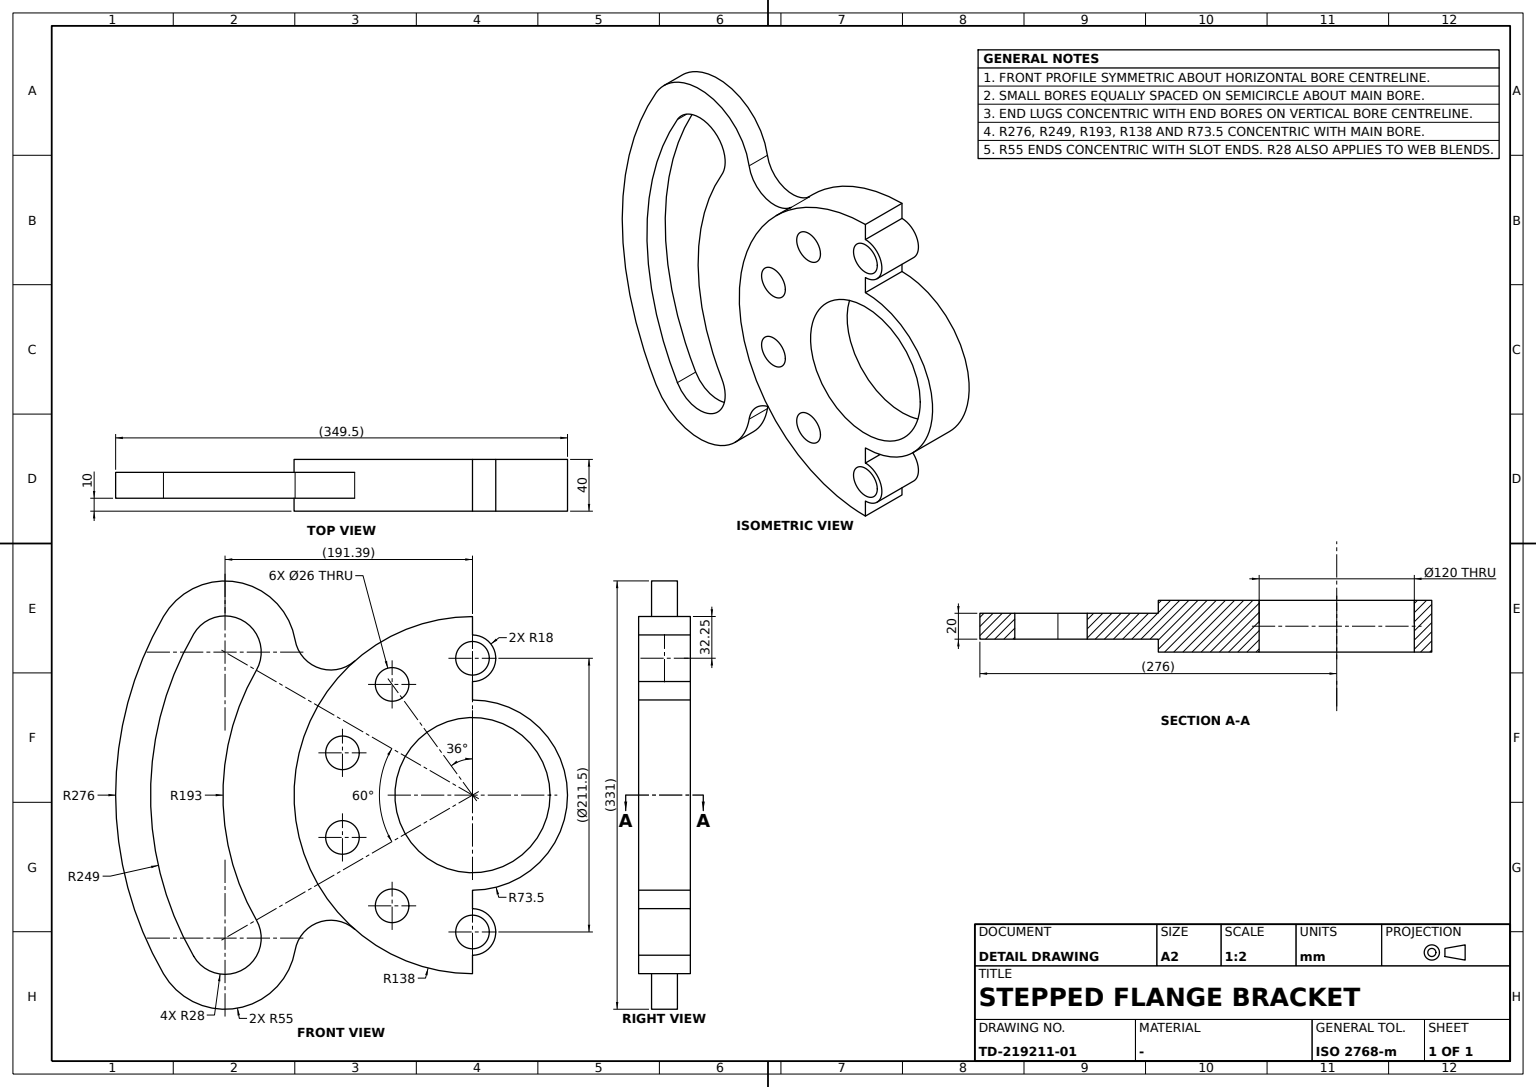
ISO-10303-21;
HEADER;
FILE_DESCRIPTION((''),'2;1');
FILE_NAME('','',(''),(''),'','','');
FILE_SCHEMA(('AUTOMOTIVE_DESIGN'));
ENDSEC;
DATA;
#1=APPLICATION_CONTEXT('');
#2=PRODUCT_CONTEXT('',#1,'mechanical');
#3=PRODUCT('','','',(#2));
#4=PRODUCT_DEFINITION_FORMATION('','',#3);
#5=PRODUCT_DEFINITION_CONTEXT('',#1,'design');
#6=PRODUCT_DEFINITION('','',#4,#5);
#7=PRODUCT_DEFINITION_SHAPE('','',#6);
#8=(LENGTH_UNIT()NAMED_UNIT(*)SI_UNIT(.MILLI.,.METRE.));
#9=(NAMED_UNIT(*)PLANE_ANGLE_UNIT()SI_UNIT($,.RADIAN.));
#10=(NAMED_UNIT(*)SI_UNIT($,.STERADIAN.)SOLID_ANGLE_UNIT());
#11=UNCERTAINTY_MEASURE_WITH_UNIT(LENGTH_MEASURE(0.005),#8,'distance_accuracy_value','');
#12=(GEOMETRIC_REPRESENTATION_CONTEXT(3)GLOBAL_UNCERTAINTY_ASSIGNED_CONTEXT((#11))GLOBAL_UNIT_ASSIGNED_CONTEXT((#8,#9,#10))REPRESENTATION_CONTEXT('',''));
#13=CARTESIAN_POINT('',(0.,-87.75,-20.));
#14=VERTEX_POINT('',#13);
#15=CARTESIAN_POINT('',(0.,-87.75,20.));
#16=VERTEX_POINT('',#15);
#17=DIRECTION('',(0.,0.,-1.));
#18=VECTOR('',#17,1000.);
#19=LINE('',#15,#18);
#20=EDGE_CURVE('',#14,#16,#19,.F.);
#21=ORIENTED_EDGE('',*,*,#20,.T.);
#22=CARTESIAN_POINT('',(0.,-123.75,20.));
#23=VERTEX_POINT('',#22);
#24=CARTESIAN_POINT('',(0.,-105.75,20.));
#25=DIRECTION('',(0.,0.,1.));
#26=DIRECTION('',(1.,0.,0.));
#27=AXIS2_PLACEMENT_3D('',#24,#25,#26);
#28=CIRCLE('',#27,18.);
#29=EDGE_CURVE('',#16,#23,#28,.F.);
#30=ORIENTED_EDGE('',*,*,#29,.T.);
#31=CARTESIAN_POINT('',(0.,-123.75,-20.));
#32=VERTEX_POINT('',#31);
#33=LINE('',#22,#18);
#34=EDGE_CURVE('',#23,#32,#33,.T.);
#35=ORIENTED_EDGE('',*,*,#34,.T.);
#36=CARTESIAN_POINT('',(0.,-105.75,-20.));
#37=AXIS2_PLACEMENT_3D('',#36,#25,#26);
#38=CIRCLE('',#37,18.);
#39=EDGE_CURVE('',#14,#32,#38,.F.);
#40=ORIENTED_EDGE('',*,*,#39,.F.);
#41=EDGE_LOOP('',(#21,#30,#35,#40));
#42=FACE_BOUND('',#41,.T.);
#43=CARTESIAN_POINT('',(0.,-105.75,0.));
#44=DIRECTION('',(0.,-1.,0.));
#45=AXIS2_PLACEMENT_3D('',#43,#17,#44);
#46=CYLINDRICAL_SURFACE('',#45,18.);
#47=ADVANCED_FACE('',(#42),#46,.T.);
#48=CARTESIAN_POINT('',(-215.640326,-124.5,10.));
#49=VERTEX_POINT('',#48);
#50=CARTESIAN_POINT('',(-215.640326,-124.5,-10.));
#51=VERTEX_POINT('',#50);
#52=CARTESIAN_POINT('',(-215.640326,-124.5,0.));
#53=VECTOR('',#25,1000.);
#54=LINE('',#52,#53);
#55=EDGE_CURVE('',#49,#51,#54,.F.);
#56=ORIENTED_EDGE('',*,*,#55,.F.);
#57=CARTESIAN_POINT('',(-167.142903,-96.5,10.));
#58=VERTEX_POINT('',#57);
#59=CARTESIAN_POINT('',(-191.391614,-110.5,10.));
#60=AXIS2_PLACEMENT_3D('',#59,#25,#26);
#61=CIRCLE('',#60,28.);
#62=EDGE_CURVE('',#49,#58,#61,.T.);
#63=ORIENTED_EDGE('',*,*,#62,.T.);
#64=CARTESIAN_POINT('',(-167.142903,-96.5,-10.));
#65=VERTEX_POINT('',#64);
#66=CARTESIAN_POINT('',(-167.142903,-96.5,0.));
#67=LINE('',#66,#53);
#68=EDGE_CURVE('',#58,#65,#67,.F.);
#69=ORIENTED_EDGE('',*,*,#68,.T.);
#70=CARTESIAN_POINT('',(-191.391614,-110.5,-10.));
#71=AXIS2_PLACEMENT_3D('',#70,#25,#26);
#72=CIRCLE('',#71,28.);
#73=EDGE_CURVE('',#51,#65,#72,.T.);
#74=ORIENTED_EDGE('',*,*,#73,.F.);
#75=EDGE_LOOP('',(#56,#63,#69,#74));
#76=FACE_BOUND('',#75,.T.);
#77=CARTESIAN_POINT('',(-191.391614,-110.5,0.));
#78=DIRECTION('',(0.,1.,0.));
#79=AXIS2_PLACEMENT_3D('',#77,#25,#78);
#80=CYLINDRICAL_SURFACE('',#79,28.);
#81=ADVANCED_FACE('',(#76),#80,.F.);
#82=CARTESIAN_POINT('',(0.,-138.,20.));
#83=VERTEX_POINT('',#82);
#84=CARTESIAN_POINT('',(0.,0.,20.));
#85=VECTOR('',#78,1000.);
#86=LINE('',#84,#85);
#87=EDGE_CURVE('',#83,#23,#86,.T.);
#88=ORIENTED_EDGE('',*,*,#87,.F.);
#89=CARTESIAN_POINT('',(0.,-138.,-20.));
#90=VERTEX_POINT('',#89);
#91=LINE('',#89,#53);
#92=EDGE_CURVE('',#90,#83,#91,.T.);
#93=ORIENTED_EDGE('',*,*,#92,.F.);
#94=CARTESIAN_POINT('',(0.,0.,-20.));
#95=LINE('',#94,#85);
#96=EDGE_CURVE('',#90,#32,#95,.T.);
#97=ORIENTED_EDGE('',*,*,#96,.T.);
#98=ORIENTED_EDGE('',*,*,#34,.F.);
#99=EDGE_LOOP('',(#88,#93,#97,#98));
#100=FACE_BOUND('',#99,.T.);
#101=CARTESIAN_POINT('',(0.,-138.,0.));
#102=AXIS2_PLACEMENT_3D('',#101,#26,#78);
#103=PLANE('',#102);
#104=ADVANCED_FACE('',(#100),#103,.T.);
#105=CARTESIAN_POINT('',(-49.15829,85.553547,20.));
#106=VERTEX_POINT('',#105);
#107=CARTESIAN_POINT('',(-62.15829,85.553547,20.));
#108=AXIS2_PLACEMENT_3D('',#107,#25,#26);
#109=CIRCLE('',#108,13.);
#110=EDGE_CURVE('',#106,#106,#109,.T.);
#111=ORIENTED_EDGE('',*,*,#110,.T.);
#112=EDGE_LOOP('',(#111));
#113=FACE_BOUND('',#112,.T.);
#114=CARTESIAN_POINT('',(-49.15829,85.553547,-20.));
#115=VERTEX_POINT('',#114);
#116=CARTESIAN_POINT('',(-62.15829,85.553547,-20.));
#117=AXIS2_PLACEMENT_3D('',#116,#25,#26);
#118=CIRCLE('',#117,13.);
#119=EDGE_CURVE('',#115,#115,#118,.T.);
#120=ORIENTED_EDGE('',*,*,#119,.F.);
#121=EDGE_LOOP('',(#120));
#122=FACE_BOUND('',#121,.T.);
#123=CARTESIAN_POINT('',(-62.15829,85.553547,-0.66));
#124=DIRECTION('',(0.809016994,0.587785252,0.));
#125=AXIS2_PLACEMENT_3D('',#123,#25,#124);
#126=CYLINDRICAL_SURFACE('',#125,13.);
#127=ADVANCED_FACE('',(#113,#122),#126,.F.);
#128=CARTESIAN_POINT('',(-91.121179,-103.638462,10.));
#129=VERTEX_POINT('',#128);
#130=CARTESIAN_POINT('',(-137.198669,-119.887477,10.));
#131=VERTEX_POINT('',#130);
#132=CARTESIAN_POINT('',(-109.609534,-124.666556,10.));
#133=AXIS2_PLACEMENT_3D('',#132,#25,#26);
#134=CIRCLE('',#133,28.);
#135=EDGE_CURVE('',#129,#131,#134,.T.);
#136=ORIENTED_EDGE('',*,*,#135,.T.);
#137=CARTESIAN_POINT('',(-137.198669,-119.887477,-10.));
#138=VERTEX_POINT('',#137);
#139=CARTESIAN_POINT('',(-137.198669,-119.887477,0.));
#140=LINE('',#139,#53);
#141=EDGE_CURVE('',#138,#131,#140,.T.);
#142=ORIENTED_EDGE('',*,*,#141,.F.);
#143=CARTESIAN_POINT('',(-91.121179,-103.638462,-10.));
#144=VERTEX_POINT('',#143);
#145=CARTESIAN_POINT('',(-109.609534,-124.666556,-10.));
#146=AXIS2_PLACEMENT_3D('',#145,#25,#26);
#147=CIRCLE('',#146,28.);
#148=EDGE_CURVE('',#144,#138,#147,.T.);
#149=ORIENTED_EDGE('',*,*,#148,.F.);
#150=CARTESIAN_POINT('',(-91.121179,-103.638462,0.));
#151=LINE('',#150,#53);
#152=EDGE_CURVE('',#144,#129,#151,.T.);
#153=ORIENTED_EDGE('',*,*,#152,.T.);
#154=EDGE_LOOP('',(#136,#142,#149,#153));
#155=FACE_BOUND('',#154,.T.);
#156=CARTESIAN_POINT('',(-109.609534,-124.666556,0.));
#157=AXIS2_PLACEMENT_3D('',#156,#25,#78);
#158=CYLINDRICAL_SURFACE('',#157,28.);
#159=ADVANCED_FACE('',(#155),#158,.F.);
#160=CARTESIAN_POINT('',(0.,-73.5,-20.));
#161=VERTEX_POINT('',#160);
#162=CARTESIAN_POINT('',(0.,73.5,-20.));
#163=VERTEX_POINT('',#162);
#164=AXIS2_PLACEMENT_3D('',#94,#25,#26);
#165=CIRCLE('',#164,73.5);
#166=EDGE_CURVE('',#161,#163,#165,.T.);
#167=ORIENTED_EDGE('',*,*,#166,.T.);
#168=CARTESIAN_POINT('',(0.,73.5,20.));
#169=VERTEX_POINT('',#168);
#170=LINE('',#162,#53);
#171=EDGE_CURVE('',#163,#169,#170,.T.);
#172=ORIENTED_EDGE('',*,*,#171,.T.);
#173=CARTESIAN_POINT('',(0.,-73.5,20.));
#174=VERTEX_POINT('',#173);
#175=AXIS2_PLACEMENT_3D('',#84,#25,#26);
#176=CIRCLE('',#175,73.5);
#177=EDGE_CURVE('',#174,#169,#176,.T.);
#178=ORIENTED_EDGE('',*,*,#177,.F.);
#179=LINE('',#160,#53);
#180=EDGE_CURVE('',#161,#174,#179,.T.);
#181=ORIENTED_EDGE('',*,*,#180,.F.);
#182=EDGE_LOOP('',(#167,#172,#178,#181));
#183=FACE_BOUND('',#182,.T.);
#184=CARTESIAN_POINT('',(0.,0.,0.));
#185=AXIS2_PLACEMENT_3D('',#184,#25,#78);
#186=CYLINDRICAL_SURFACE('',#185,73.5);
#187=ADVANCED_FACE('',(#183),#186,.T.);
#188=CARTESIAN_POINT('',(-87.574227,-32.678547,20.));
#189=VERTEX_POINT('',#188);
#190=CARTESIAN_POINT('',(-100.574227,-32.678547,20.));
#191=AXIS2_PLACEMENT_3D('',#190,#25,#26);
#192=CIRCLE('',#191,13.);
#193=EDGE_CURVE('',#189,#189,#192,.T.);
#194=ORIENTED_EDGE('',*,*,#193,.T.);
#195=EDGE_LOOP('',(#194));
#196=FACE_BOUND('',#195,.T.);
#197=CARTESIAN_POINT('',(-87.574227,-32.678547,-20.));
#198=VERTEX_POINT('',#197);
#199=CARTESIAN_POINT('',(-100.574227,-32.678547,-20.));
#200=AXIS2_PLACEMENT_3D('',#199,#25,#26);
#201=CIRCLE('',#200,13.);
#202=EDGE_CURVE('',#198,#198,#201,.T.);
#203=ORIENTED_EDGE('',*,*,#202,.F.);
#204=EDGE_LOOP('',(#203));
#205=FACE_BOUND('',#204,.T.);
#206=CARTESIAN_POINT('',(-100.574227,-32.678547,-0.66));
#207=DIRECTION('',(-0.309016994,0.951056516,0.));
#208=AXIS2_PLACEMENT_3D('',#206,#25,#207);
#209=CYLINDRICAL_SURFACE('',#208,13.);
#210=ADVANCED_FACE('',(#196,#205),#209,.F.);
#211=CARTESIAN_POINT('',(-215.640326,124.5,10.));
#212=VERTEX_POINT('',#211);
#213=CARTESIAN_POINT('',(0.,0.,10.));
#214=AXIS2_PLACEMENT_3D('',#213,#25,#26);
#215=CIRCLE('',#214,249.);
#216=EDGE_CURVE('',#212,#49,#215,.T.);
#217=ORIENTED_EDGE('',*,*,#216,.T.);
#218=ORIENTED_EDGE('',*,*,#55,.T.);
#219=CARTESIAN_POINT('',(-215.640326,124.5,-10.));
#220=VERTEX_POINT('',#219);
#221=CARTESIAN_POINT('',(0.,0.,-10.));
#222=AXIS2_PLACEMENT_3D('',#221,#25,#26);
#223=CIRCLE('',#222,249.);
#224=EDGE_CURVE('',#220,#51,#223,.T.);
#225=ORIENTED_EDGE('',*,*,#224,.F.);
#226=CARTESIAN_POINT('',(-215.640326,124.5,0.));
#227=LINE('',#226,#53);
#228=EDGE_CURVE('',#212,#220,#227,.F.);
#229=ORIENTED_EDGE('',*,*,#228,.F.);
#230=EDGE_LOOP('',(#217,#218,#225,#229));
#231=FACE_BOUND('',#230,.T.);
#232=CYLINDRICAL_SURFACE('',#185,249.);
#233=ADVANCED_FACE('',(#231),#232,.F.);
#234=CARTESIAN_POINT('',(-167.142903,96.5,-10.));
#235=VERTEX_POINT('',#234);
#236=CIRCLE('',#222,193.);
#237=EDGE_CURVE('',#235,#65,#236,.T.);
#238=ORIENTED_EDGE('',*,*,#237,.T.);
#239=ORIENTED_EDGE('',*,*,#68,.F.);
#240=CARTESIAN_POINT('',(-167.142903,96.5,10.));
#241=VERTEX_POINT('',#240);
#242=CIRCLE('',#214,193.);
#243=EDGE_CURVE('',#241,#58,#242,.T.);
#244=ORIENTED_EDGE('',*,*,#243,.F.);
#245=CARTESIAN_POINT('',(-167.142903,96.5,0.));
#246=LINE('',#245,#53);
#247=EDGE_CURVE('',#241,#235,#246,.F.);
#248=ORIENTED_EDGE('',*,*,#247,.T.);
#249=EDGE_LOOP('',(#238,#239,#244,#248));
#250=FACE_BOUND('',#249,.T.);
#251=CYLINDRICAL_SURFACE('',#185,193.);
#252=ADVANCED_FACE('',(#250),#251,.T.);
#253=CARTESIAN_POINT('',(60.,0.,20.));
#254=VERTEX_POINT('',#253);
#255=CIRCLE('',#175,60.);
#256=EDGE_CURVE('',#254,#254,#255,.T.);
#257=ORIENTED_EDGE('',*,*,#256,.T.);
#258=EDGE_LOOP('',(#257));
#259=FACE_BOUND('',#258,.T.);
#260=CARTESIAN_POINT('',(60.,0.,-20.));
#261=VERTEX_POINT('',#260);
#262=CIRCLE('',#164,60.);
#263=EDGE_CURVE('',#261,#261,#262,.T.);
#264=ORIENTED_EDGE('',*,*,#263,.F.);
#265=EDGE_LOOP('',(#264));
#266=FACE_BOUND('',#265,.T.);
#267=CYLINDRICAL_SURFACE('',#185,60.);
#268=ADVANCED_FACE('',(#259,#266),#267,.F.);
#269=CARTESIAN_POINT('',(0.,87.75,20.));
#270=VERTEX_POINT('',#269);
#271=CARTESIAN_POINT('',(0.,123.75,20.));
#272=VERTEX_POINT('',#271);
#273=CARTESIAN_POINT('',(0.,105.75,20.));
#274=AXIS2_PLACEMENT_3D('',#273,#25,#26);
#275=CIRCLE('',#274,18.);
#276=EDGE_CURVE('',#270,#272,#275,.T.);
#277=ORIENTED_EDGE('',*,*,#276,.F.);
#278=CARTESIAN_POINT('',(0.,87.75,-20.));
#279=VERTEX_POINT('',#278);
#280=LINE('',#269,#53);
#281=EDGE_CURVE('',#279,#270,#280,.T.);
#282=ORIENTED_EDGE('',*,*,#281,.F.);
#283=CARTESIAN_POINT('',(0.,123.75,-20.));
#284=VERTEX_POINT('',#283);
#285=CARTESIAN_POINT('',(0.,105.75,-20.));
#286=AXIS2_PLACEMENT_3D('',#285,#25,#26);
#287=CIRCLE('',#286,18.);
#288=EDGE_CURVE('',#279,#284,#287,.T.);
#289=ORIENTED_EDGE('',*,*,#288,.T.);
#290=LINE('',#271,#53);
#291=EDGE_CURVE('',#272,#284,#290,.F.);
#292=ORIENTED_EDGE('',*,*,#291,.F.);
#293=EDGE_LOOP('',(#277,#282,#289,#292));
#294=FACE_BOUND('',#293,.T.);
#295=CARTESIAN_POINT('',(0.,105.75,0.));
#296=AXIS2_PLACEMENT_3D('',#295,#25,#78);
#297=CYLINDRICAL_SURFACE('',#296,18.);
#298=ADVANCED_FACE('',(#294),#297,.T.);
#299=CARTESIAN_POINT('',(-87.574227,32.678547,-20.));
#300=VERTEX_POINT('',#299);
#301=CARTESIAN_POINT('',(-100.574227,32.678547,-20.));
#302=AXIS2_PLACEMENT_3D('',#301,#25,#26);
#303=CIRCLE('',#302,13.);
#304=EDGE_CURVE('',#300,#300,#303,.T.);
#305=ORIENTED_EDGE('',*,*,#304,.F.);
#306=EDGE_LOOP('',(#305));
#307=FACE_BOUND('',#306,.T.);
#308=CARTESIAN_POINT('',(-87.574227,32.678547,20.));
#309=VERTEX_POINT('',#308);
#310=CARTESIAN_POINT('',(-100.574227,32.678547,20.));
#311=AXIS2_PLACEMENT_3D('',#310,#25,#26);
#312=CIRCLE('',#311,13.);
#313=EDGE_CURVE('',#309,#309,#312,.T.);
#314=ORIENTED_EDGE('',*,*,#313,.T.);
#315=EDGE_LOOP('',(#314));
#316=FACE_BOUND('',#315,.T.);
#317=CARTESIAN_POINT('',(-100.574227,32.678547,-0.66));
#318=DIRECTION('',(0.309016994,0.951056516,0.));
#319=AXIS2_PLACEMENT_3D('',#317,#25,#318);
#320=CYLINDRICAL_SURFACE('',#319,13.);
#321=ADVANCED_FACE('',(#307,#316),#320,.F.);
#322=ORIENTED_EDGE('',*,*,#20,.F.);
#323=EDGE_CURVE('',#14,#161,#95,.T.);
#324=ORIENTED_EDGE('',*,*,#323,.T.);
#325=ORIENTED_EDGE('',*,*,#180,.T.);
#326=EDGE_CURVE('',#16,#174,#86,.T.);
#327=ORIENTED_EDGE('',*,*,#326,.F.);
#328=EDGE_LOOP('',(#322,#324,#325,#327));
#329=FACE_BOUND('',#328,.T.);
#330=ADVANCED_FACE('',(#329),#103,.T.);
#331=CARTESIAN_POINT('',(13.,105.75,-20.));
#332=VERTEX_POINT('',#331);
#333=CIRCLE('',#286,13.);
#334=EDGE_CURVE('',#332,#332,#333,.T.);
#335=ORIENTED_EDGE('',*,*,#334,.F.);
#336=EDGE_LOOP('',(#335));
#337=FACE_BOUND('',#336,.T.);
#338=CARTESIAN_POINT('',(13.,105.75,20.));
#339=VERTEX_POINT('',#338);
#340=CIRCLE('',#274,13.);
#341=EDGE_CURVE('',#339,#339,#340,.T.);
#342=ORIENTED_EDGE('',*,*,#341,.T.);
#343=EDGE_LOOP('',(#342));
#344=FACE_BOUND('',#343,.T.);
#345=CARTESIAN_POINT('',(0.,105.75,-0.66));
#346=AXIS2_PLACEMENT_3D('',#345,#25,#26);
#347=CYLINDRICAL_SURFACE('',#346,13.);
#348=ADVANCED_FACE('',(#337,#344),#347,.F.);
#349=CARTESIAN_POINT('',(0.,138.,20.));
#350=VERTEX_POINT('',#349);
#351=EDGE_CURVE('',#272,#350,#86,.T.);
#352=ORIENTED_EDGE('',*,*,#351,.F.);
#353=ORIENTED_EDGE('',*,*,#291,.T.);
#354=CARTESIAN_POINT('',(0.,138.,-20.));
#355=VERTEX_POINT('',#354);
#356=EDGE_CURVE('',#284,#355,#95,.T.);
#357=ORIENTED_EDGE('',*,*,#356,.T.);
#358=LINE('',#354,#53);
#359=EDGE_CURVE('',#355,#350,#358,.T.);
#360=ORIENTED_EDGE('',*,*,#359,.T.);
#361=EDGE_LOOP('',(#352,#353,#357,#360));
#362=FACE_BOUND('',#361,.T.);
#363=ADVANCED_FACE('',(#362),#103,.T.);
#364=CARTESIAN_POINT('',(-239.023011,138.,-10.));
#365=VERTEX_POINT('',#364);
#366=CARTESIAN_POINT('',(-239.023011,138.,10.));
#367=VERTEX_POINT('',#366);
#368=CARTESIAN_POINT('',(-239.023011,138.,0.));
#369=LINE('',#368,#53);
#370=EDGE_CURVE('',#365,#367,#369,.T.);
#371=ORIENTED_EDGE('',*,*,#370,.F.);
#372=CARTESIAN_POINT('',(-239.023011,-138.,-10.));
#373=VERTEX_POINT('',#372);
#374=CIRCLE('',#222,276.);
#375=EDGE_CURVE('',#365,#373,#374,.T.);
#376=ORIENTED_EDGE('',*,*,#375,.T.);
#377=CARTESIAN_POINT('',(-239.023011,-138.,10.));
#378=VERTEX_POINT('',#377);
#379=CARTESIAN_POINT('',(-239.023011,-138.,0.));
#380=LINE('',#379,#53);
#381=EDGE_CURVE('',#373,#378,#380,.T.);
#382=ORIENTED_EDGE('',*,*,#381,.T.);
#383=CIRCLE('',#214,276.);
#384=EDGE_CURVE('',#367,#378,#383,.T.);
#385=ORIENTED_EDGE('',*,*,#384,.F.);
#386=EDGE_LOOP('',(#371,#376,#382,#385));
#387=FACE_BOUND('',#386,.T.);
#388=CYLINDRICAL_SURFACE('',#185,276.);
#389=ADVANCED_FACE('',(#387),#388,.T.);
#390=CIRCLE('',#60,55.);
#391=EDGE_CURVE('',#378,#131,#390,.T.);
#392=ORIENTED_EDGE('',*,*,#391,.F.);
#393=ORIENTED_EDGE('',*,*,#381,.F.);
#394=CIRCLE('',#71,55.);
#395=EDGE_CURVE('',#373,#138,#394,.T.);
#396=ORIENTED_EDGE('',*,*,#395,.T.);
#397=ORIENTED_EDGE('',*,*,#141,.T.);
#398=EDGE_LOOP('',(#392,#393,#396,#397));
#399=FACE_BOUND('',#398,.T.);
#400=CYLINDRICAL_SURFACE('',#79,55.);
#401=ADVANCED_FACE('',(#399),#400,.T.);
#402=ORIENTED_EDGE('',*,*,#243,.T.);
#403=ORIENTED_EDGE('',*,*,#62,.F.);
#404=ORIENTED_EDGE('',*,*,#216,.F.);
#405=CARTESIAN_POINT('',(-191.391614,110.5,10.));
#406=AXIS2_PLACEMENT_3D('',#405,#25,#26);
#407=CIRCLE('',#406,28.);
#408=EDGE_CURVE('',#241,#212,#407,.T.);
#409=ORIENTED_EDGE('',*,*,#408,.F.);
#410=EDGE_LOOP('',(#402,#403,#404,#409));
#411=FACE_BOUND('',#410,.T.);
#412=CARTESIAN_POINT('',(-91.121179,103.638462,10.));
#413=VERTEX_POINT('',#412);
#414=CIRCLE('',#214,138.);
#415=EDGE_CURVE('',#413,#129,#414,.T.);
#416=ORIENTED_EDGE('',*,*,#415,.F.);
#417=CARTESIAN_POINT('',(-137.198669,119.887477,10.));
#418=VERTEX_POINT('',#417);
#419=CARTESIAN_POINT('',(-109.609534,124.666556,10.));
#420=AXIS2_PLACEMENT_3D('',#419,#25,#26);
#421=CIRCLE('',#420,28.);
#422=EDGE_CURVE('',#418,#413,#421,.T.);
#423=ORIENTED_EDGE('',*,*,#422,.F.);
#424=CIRCLE('',#406,55.);
#425=EDGE_CURVE('',#418,#367,#424,.T.);
#426=ORIENTED_EDGE('',*,*,#425,.T.);
#427=ORIENTED_EDGE('',*,*,#384,.T.);
#428=ORIENTED_EDGE('',*,*,#391,.T.);
#429=ORIENTED_EDGE('',*,*,#135,.F.);
#430=EDGE_LOOP('',(#416,#423,#426,#427,#428,#429));
#431=FACE_BOUND('',#430,.T.);
#432=AXIS2_PLACEMENT_3D('',#213,#25,#78);
#433=PLANE('',#432);
#434=ADVANCED_FACE('',(#411,#431),#433,.T.);
#435=CARTESIAN_POINT('',(-49.15829,-85.553547,-20.));
#436=VERTEX_POINT('',#435);
#437=CARTESIAN_POINT('',(-62.15829,-85.553547,-20.));
#438=AXIS2_PLACEMENT_3D('',#437,#25,#26);
#439=CIRCLE('',#438,13.);
#440=EDGE_CURVE('',#436,#436,#439,.T.);
#441=ORIENTED_EDGE('',*,*,#440,.F.);
#442=EDGE_LOOP('',(#441));
#443=FACE_BOUND('',#442,.T.);
#444=CARTESIAN_POINT('',(-49.15829,-85.553547,20.));
#445=VERTEX_POINT('',#444);
#446=CARTESIAN_POINT('',(-62.15829,-85.553547,20.));
#447=AXIS2_PLACEMENT_3D('',#446,#25,#26);
#448=CIRCLE('',#447,13.);
#449=EDGE_CURVE('',#445,#445,#448,.T.);
#450=ORIENTED_EDGE('',*,*,#449,.T.);
#451=EDGE_LOOP('',(#450));
#452=FACE_BOUND('',#451,.T.);
#453=CARTESIAN_POINT('',(-62.15829,-85.553547,-0.66));
#454=DIRECTION('',(-0.809016994,0.587785252,0.));
#455=AXIS2_PLACEMENT_3D('',#453,#25,#454);
#456=CYLINDRICAL_SURFACE('',#455,13.);
#457=ADVANCED_FACE('',(#443,#452),#456,.F.);
#458=ORIENTED_EDGE('',*,*,#422,.T.);
#459=CARTESIAN_POINT('',(-91.121179,103.638462,-10.));
#460=VERTEX_POINT('',#459);
#461=CARTESIAN_POINT('',(-91.121179,103.638462,0.));
#462=LINE('',#461,#53);
#463=EDGE_CURVE('',#460,#413,#462,.T.);
#464=ORIENTED_EDGE('',*,*,#463,.F.);
#465=CARTESIAN_POINT('',(-137.198669,119.887477,-10.));
#466=VERTEX_POINT('',#465);
#467=CARTESIAN_POINT('',(-109.609534,124.666556,-10.));
#468=AXIS2_PLACEMENT_3D('',#467,#25,#26);
#469=CIRCLE('',#468,28.);
#470=EDGE_CURVE('',#466,#460,#469,.T.);
#471=ORIENTED_EDGE('',*,*,#470,.F.);
#472=CARTESIAN_POINT('',(-137.198669,119.887477,0.));
#473=LINE('',#472,#53);
#474=EDGE_CURVE('',#466,#418,#473,.T.);
#475=ORIENTED_EDGE('',*,*,#474,.T.);
#476=EDGE_LOOP('',(#458,#464,#471,#475));
#477=FACE_BOUND('',#476,.T.);
#478=CARTESIAN_POINT('',(-109.609534,124.666556,0.));
#479=AXIS2_PLACEMENT_3D('',#478,#25,#78);
#480=CYLINDRICAL_SURFACE('',#479,28.);
#481=ADVANCED_FACE('',(#477),#480,.F.);
#482=EDGE_CURVE('',#169,#270,#86,.T.);
#483=ORIENTED_EDGE('',*,*,#482,.F.);
#484=ORIENTED_EDGE('',*,*,#171,.F.);
#485=EDGE_CURVE('',#163,#279,#95,.T.);
#486=ORIENTED_EDGE('',*,*,#485,.T.);
#487=ORIENTED_EDGE('',*,*,#281,.T.);
#488=EDGE_LOOP('',(#483,#484,#486,#487));
#489=FACE_BOUND('',#488,.T.);
#490=ADVANCED_FACE('',(#489),#103,.T.);
#491=CIRCLE('',#164,138.);
#492=EDGE_CURVE('',#355,#90,#491,.T.);
#493=ORIENTED_EDGE('',*,*,#492,.T.);
#494=ORIENTED_EDGE('',*,*,#92,.T.);
#495=CIRCLE('',#175,138.);
#496=EDGE_CURVE('',#350,#83,#495,.T.);
#497=ORIENTED_EDGE('',*,*,#496,.F.);
#498=ORIENTED_EDGE('',*,*,#359,.F.);
#499=EDGE_LOOP('',(#493,#494,#497,#498));
#500=FACE_BOUND('',#499,.T.);
#501=ORIENTED_EDGE('',*,*,#463,.T.);
#502=ORIENTED_EDGE('',*,*,#415,.T.);
#503=ORIENTED_EDGE('',*,*,#152,.F.);
#504=CIRCLE('',#222,138.);
#505=EDGE_CURVE('',#460,#144,#504,.T.);
#506=ORIENTED_EDGE('',*,*,#505,.F.);
#507=EDGE_LOOP('',(#501,#502,#503,#506));
#508=FACE_BOUND('',#507,.T.);
#509=CYLINDRICAL_SURFACE('',#185,138.);
#510=ADVANCED_FACE('',(#500,#508),#509,.T.);
#511=ORIENTED_EDGE('',*,*,#408,.T.);
#512=ORIENTED_EDGE('',*,*,#228,.T.);
#513=CARTESIAN_POINT('',(-191.391614,110.5,-10.));
#514=AXIS2_PLACEMENT_3D('',#513,#25,#26);
#515=CIRCLE('',#514,28.);
#516=EDGE_CURVE('',#235,#220,#515,.T.);
#517=ORIENTED_EDGE('',*,*,#516,.F.);
#518=ORIENTED_EDGE('',*,*,#247,.F.);
#519=EDGE_LOOP('',(#511,#512,#517,#518));
#520=FACE_BOUND('',#519,.T.);
#521=CARTESIAN_POINT('',(-191.391614,110.5,0.));
#522=AXIS2_PLACEMENT_3D('',#521,#25,#78);
#523=CYLINDRICAL_SURFACE('',#522,28.);
#524=ADVANCED_FACE('',(#520),#523,.F.);
#525=ORIENTED_EDGE('',*,*,#474,.F.);
#526=CIRCLE('',#514,55.);
#527=EDGE_CURVE('',#466,#365,#526,.T.);
#528=ORIENTED_EDGE('',*,*,#527,.T.);
#529=ORIENTED_EDGE('',*,*,#370,.T.);
#530=ORIENTED_EDGE('',*,*,#425,.F.);
#531=EDGE_LOOP('',(#525,#528,#529,#530));
#532=FACE_BOUND('',#531,.T.);
#533=CYLINDRICAL_SURFACE('',#522,55.);
#534=ADVANCED_FACE('',(#532),#533,.T.);
#535=ORIENTED_EDGE('',*,*,#341,.F.);
#536=EDGE_LOOP('',(#535));
#537=FACE_BOUND('',#536,.T.);
#538=ORIENTED_EDGE('',*,*,#256,.F.);
#539=EDGE_LOOP('',(#538));
#540=FACE_BOUND('',#539,.T.);
#541=ORIENTED_EDGE('',*,*,#351,.T.);
#542=ORIENTED_EDGE('',*,*,#496,.T.);
#543=ORIENTED_EDGE('',*,*,#87,.T.);
#544=ORIENTED_EDGE('',*,*,#29,.F.);
#545=ORIENTED_EDGE('',*,*,#326,.T.);
#546=ORIENTED_EDGE('',*,*,#177,.T.);
#547=ORIENTED_EDGE('',*,*,#482,.T.);
#548=ORIENTED_EDGE('',*,*,#276,.T.);
#549=EDGE_LOOP('',(#541,#542,#543,#544,#545,#546,#547,#548));
#550=FACE_BOUND('',#549,.T.);
#551=ORIENTED_EDGE('',*,*,#449,.F.);
#552=EDGE_LOOP('',(#551));
#553=FACE_BOUND('',#552,.T.);
#554=CARTESIAN_POINT('',(13.,-105.75,20.));
#555=VERTEX_POINT('',#554);
#556=CIRCLE('',#27,13.);
#557=EDGE_CURVE('',#555,#555,#556,.T.);
#558=ORIENTED_EDGE('',*,*,#557,.F.);
#559=EDGE_LOOP('',(#558));
#560=FACE_BOUND('',#559,.T.);
#561=ORIENTED_EDGE('',*,*,#193,.F.);
#562=EDGE_LOOP('',(#561));
#563=FACE_BOUND('',#562,.T.);
#564=ORIENTED_EDGE('',*,*,#313,.F.);
#565=EDGE_LOOP('',(#564));
#566=FACE_BOUND('',#565,.T.);
#567=ORIENTED_EDGE('',*,*,#110,.F.);
#568=EDGE_LOOP('',(#567));
#569=FACE_BOUND('',#568,.T.);
#570=AXIS2_PLACEMENT_3D('',#84,#25,#78);
#571=PLANE('',#570);
#572=ADVANCED_FACE('',(#537,#540,#550,#553,#560,#563,#566,#569),#571,.T.);
#573=CARTESIAN_POINT('',(13.,-105.75,-20.));
#574=VERTEX_POINT('',#573);
#575=CIRCLE('',#37,13.);
#576=EDGE_CURVE('',#574,#574,#575,.T.);
#577=ORIENTED_EDGE('',*,*,#576,.F.);
#578=EDGE_LOOP('',(#577));
#579=FACE_BOUND('',#578,.T.);
#580=ORIENTED_EDGE('',*,*,#557,.T.);
#581=EDGE_LOOP('',(#580));
#582=FACE_BOUND('',#581,.T.);
#583=CARTESIAN_POINT('',(0.,-105.75,-0.66));
#584=DIRECTION('',(-1.,0.,0.));
#585=AXIS2_PLACEMENT_3D('',#583,#25,#584);
#586=CYLINDRICAL_SURFACE('',#585,13.);
#587=ADVANCED_FACE('',(#579,#582),#586,.F.);
#588=ORIENTED_EDGE('',*,*,#288,.F.);
#589=ORIENTED_EDGE('',*,*,#485,.F.);
#590=ORIENTED_EDGE('',*,*,#166,.F.);
#591=ORIENTED_EDGE('',*,*,#323,.F.);
#592=ORIENTED_EDGE('',*,*,#39,.T.);
#593=ORIENTED_EDGE('',*,*,#96,.F.);
#594=ORIENTED_EDGE('',*,*,#492,.F.);
#595=ORIENTED_EDGE('',*,*,#356,.F.);
#596=EDGE_LOOP('',(#588,#589,#590,#591,#592,#593,#594,#595));
#597=FACE_BOUND('',#596,.T.);
#598=ORIENTED_EDGE('',*,*,#263,.T.);
#599=EDGE_LOOP('',(#598));
#600=FACE_BOUND('',#599,.T.);
#601=ORIENTED_EDGE('',*,*,#440,.T.);
#602=EDGE_LOOP('',(#601));
#603=FACE_BOUND('',#602,.T.);
#604=ORIENTED_EDGE('',*,*,#119,.T.);
#605=EDGE_LOOP('',(#604));
#606=FACE_BOUND('',#605,.T.);
#607=ORIENTED_EDGE('',*,*,#576,.T.);
#608=EDGE_LOOP('',(#607));
#609=FACE_BOUND('',#608,.T.);
#610=ORIENTED_EDGE('',*,*,#202,.T.);
#611=EDGE_LOOP('',(#610));
#612=FACE_BOUND('',#611,.T.);
#613=ORIENTED_EDGE('',*,*,#334,.T.);
#614=EDGE_LOOP('',(#613));
#615=FACE_BOUND('',#614,.T.);
#616=ORIENTED_EDGE('',*,*,#304,.T.);
#617=EDGE_LOOP('',(#616));
#618=FACE_BOUND('',#617,.T.);
#619=AXIS2_PLACEMENT_3D('',#94,#25,#78);
#620=PLANE('',#619);
#621=ADVANCED_FACE('',(#597,#600,#603,#606,#609,#612,#615,#618),#620,.F.);
#622=ORIENTED_EDGE('',*,*,#375,.F.);
#623=ORIENTED_EDGE('',*,*,#527,.F.);
#624=ORIENTED_EDGE('',*,*,#470,.T.);
#625=ORIENTED_EDGE('',*,*,#505,.T.);
#626=ORIENTED_EDGE('',*,*,#148,.T.);
#627=ORIENTED_EDGE('',*,*,#395,.F.);
#628=EDGE_LOOP('',(#622,#623,#624,#625,#626,#627));
#629=FACE_BOUND('',#628,.T.);
#630=ORIENTED_EDGE('',*,*,#224,.T.);
#631=ORIENTED_EDGE('',*,*,#73,.T.);
#632=ORIENTED_EDGE('',*,*,#237,.F.);
#633=ORIENTED_EDGE('',*,*,#516,.T.);
#634=EDGE_LOOP('',(#630,#631,#632,#633));
#635=FACE_BOUND('',#634,.T.);
#636=AXIS2_PLACEMENT_3D('',#221,#25,#78);
#637=PLANE('',#636);
#638=ADVANCED_FACE('',(#629,#635),#637,.F.);
#639=CLOSED_SHELL('',(#47,#81,#104,#127,#159,#187,#210,#233,#252,#268,#298,#321,#330,#348,#363,#389,#401,#434,#457,#481,#490,#510,#524,#534,#572,#587,#621,#638));
#640=MANIFOLD_SOLID_BREP('',#639);
#641=ADVANCED_BREP_SHAPE_REPRESENTATION('',(#640),#12);
#642=SHAPE_DEFINITION_REPRESENTATION(#7,#641);
ENDSEC;
END-ISO-10303-21;
